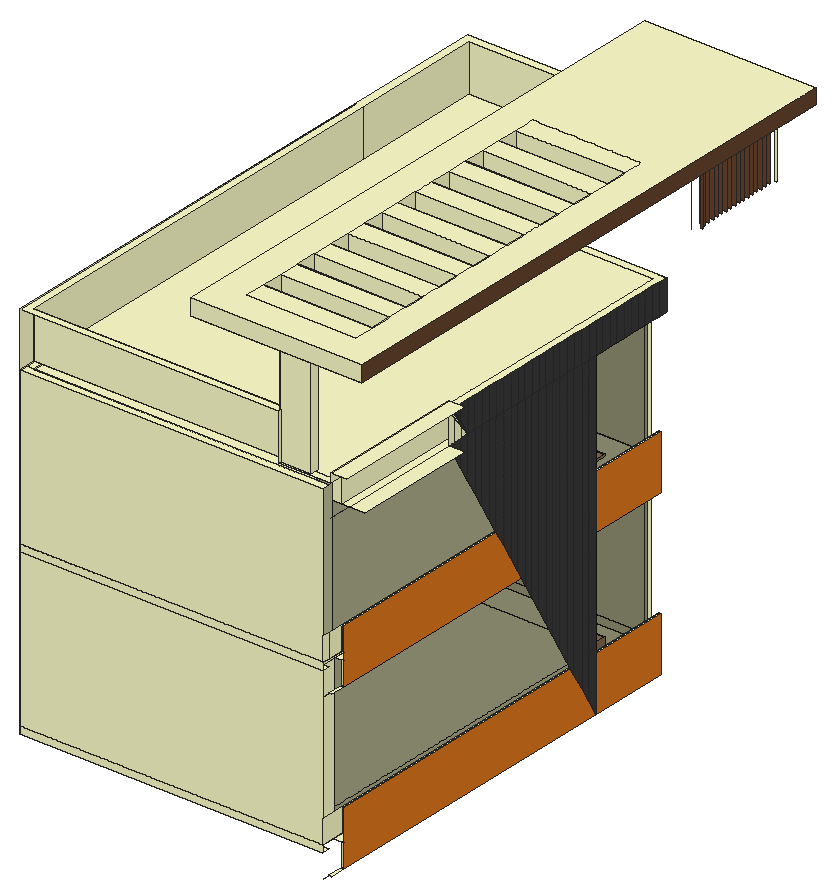
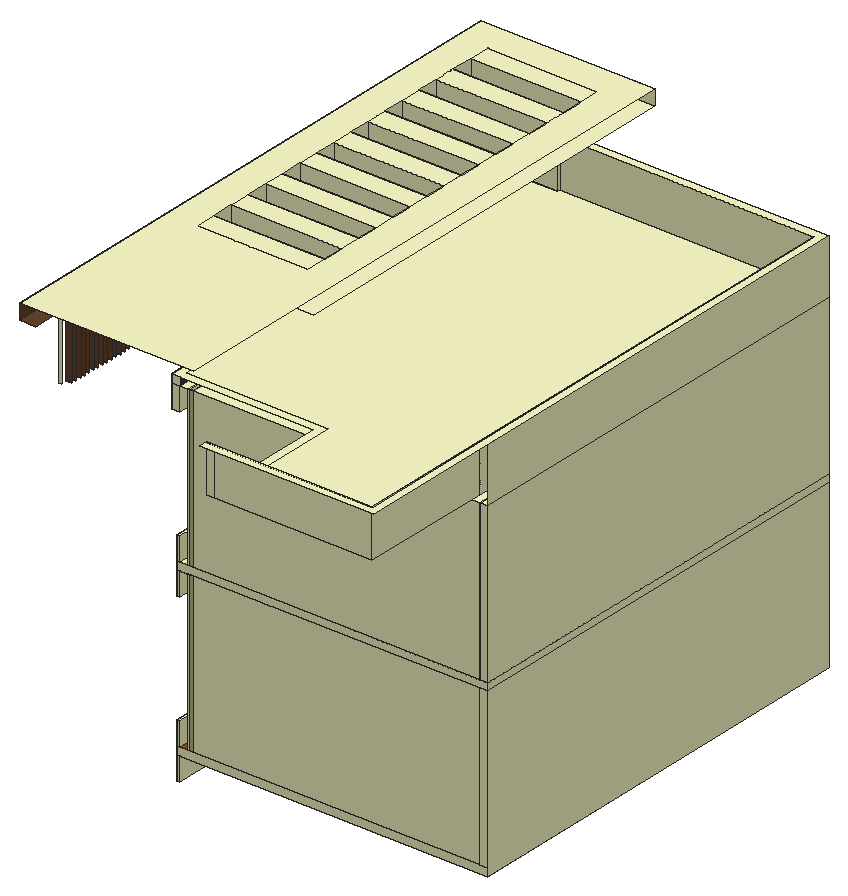
# SketchUp Ruby script. Lengths in inches.
U = 1.inch
M = Sketchup.active_model
def pt(a) = Geom::Point3d.new(a.map { |v| v * U })
def face(e, loops, mat)
  f = e.add_face(loops[0].map { |a| pt(a) })
  loops[1..].each { |l| e.add_face(l.map { |a| pt(a) }).erase! }
  f.material = f.back_material = mat if mat
  f
end
# faces: each face lists its corners as indices into pts; further lists are holes
def faces(e, pts, list, mat = nil) = list.each { |f| face(e, (f[0].is_a?(Array) ? f : [f]).map { |l| l.map { |i| pts[i] } }, mat) }
# xy, xz, yz: faces in a plane at the given z, y or x. An outline is a flat list of corners, or four numbers for a rectangle; further outlines are holes
def ring(l) = l.size == 4 ? [[l[0], l[1]], [l[2], l[1]], [l[2], l[3]], [l[0], l[3]]] : l.each_slice(2).to_a
def flat(e, list, mat, &to3) = list.each { |f| face(e, (f[0].is_a?(Array) ? f : [f]).map { |l| ring(l).map { |u, v| to3.(u, v) } }, mat) }
def xy(e, z, list, mat = nil) = flat(e, list, mat) { |x, y| [x, y, z] }
def xz(e, y, list, mat = nil) = flat(e, list, mat) { |x, z| [x, y, z] }
def yz(e, x, list, mat = nil) = flat(e, list, mat) { |y, z| [x, y, z] }
def lines(e, pts, list) = list.each { |a, b| e.add_line(pt(pts[a]), pt(pts[b])) }
# prism: a flat outline (further loops are holes) pulled along v
def prism(e, loops, v, mat = nil)
  f = face(e, loops, mat); d = Geom::Vector3d.new(v.map { |x| x * U })
  f.pushpull(f.normal.samedirection?(d) ? d.length : -d.length)
end
def box(e, o, s, mat = nil) = prism(e, [[o, [o[0] + s[0], o[1], o[2]], [o[0] + s[0], o[1] + s[1], o[2]], [o[0], o[1] + s[1], o[2]]]], [0, 0, s[2]], mat)
def at(x, y, z, deg = 0) = Geom::Transformation.translation(pt([x, y, z])) * Geom::Transformation.rotation(ORIGIN, Z_AXIS, deg.degrees)
def axes(o, x, y, z) = Geom::Transformation.new([*x, 0, *y, 0, *z, 0, *pt(o).to_a, 1])
def part(name) = M.definitions.add(name)
# library, detail: a bought-in or finely detailed component or shape, given as its bounding box
def library(name, o, s) = part(name).tap { |d| box(d.entities, o, s) }
def detail(e, o, s) = box(e.add_group.entities, o, s)
def put(e, d, t, mat = nil) = e.add_instance(d, t).tap { |i| i.material = mat if mat }
def group(e, t, mat = nil) = e.add_group.tap { |g| g.transformation = t; g.material = mat if mat }.entities
root = M.entities
M.materials.add("Brick_Common_Bond_2K").color = [226, 121, 29]
M.materials.add("E01_Mint_Frost").color = [255, 255, 204]
M.materials.add("Glass_Safety_01").color = [0, 0, 0]
M.materials["Glass_Safety_01"].alpha = 0.25
M.materials.add("M07_Charcoal_Gleam").color = [58, 58, 58]
M.materials.add("Wood_Veneer_15_1K").color = [103, 69, 45]
c1 = library("Sphere Light\#7",[-4.28,-4.28,-4.28],[8.56,8.56,8.56])
c2 = library("Sphere Light\#5",[-3.78,-3.78,-3.78],[7.56,7.56,7.56])
c3 = library("Sphere Light\#6",[-3.67,-3.67,-3.67],[7.34,7.34,7.34])
c4 = library("Sphere Light\#4",[-3.65,-3.65,-3.65],[7.3,7.3,7.3])
c5 = part("Group\#3")
box(c5.entities,[0,0,0],[3,318,120])
c6 = library("Sphere Light\#3",[-3.21,-3.21,-3.21],[6.42,6.42,6.42])
c7 = library("Sphere Light\#2",[-4.11,-4.11,-4.11],[8.22,8.22,8.22])
c8 = library("Sphere Light\#1",[-3.65,-3.65,-3.65],[7.3,7.3,7.3])
c9 = library("Sphere Light",[-3.57,-3.57,-3.57],[7.14,7.14,7.14])
xy(root,492,[[469.07,81.71,471.07,93.71],[469.07,93.71,471.07,399.71]],"E01_Mint_Frost")
xy(root,510,[[235.07,75.71,469.07,81.71],[235.07,81.71,241.07,399.71],[[241.07,81.71,463.07,399.71],[439.31,101.72,440.34,101.92,441.27,102.375,442.0625,103.06,442.65,103.92,442.99,104.91,443.07,105.95,442.87,106.98,442.41,107.92,441.73,108.7,440.87,109.29,439.88,109.63,439.07,109.69,439.07,371.73,439.24,371.72,440.27,371.9,441.22,372.34,442.02,373.01,442.62,373.86,442.98,374.84,443.07,375.88,442.89,376.91,442.45,377.86,441.78,378.66,440.93,379.26,439.95,379.62,438.91,379.71,437.88,379.53,436.93,379.09,436.13,378.42,435.53,377.57,435.17,376.59,435.09,375.71,269.07,375.71,268.9375,376.75,268.54,377.71,267.9,378.54,267.07,379.18,266.11,379.58,265.07,379.71,264.04,379.58,263.07,379.18,262.25,378.54,261.61,377.71,261.21,376.75,261.07,375.71,261.21,374.68,261.61,373.71,262.25,372.89,263.07,372.25,264.04,371.85,265.07,371.71,265.07,109.68,264.43,109.66,263.43,109.36,262.54,108.8125,261.83,108.05,261.33,107.13,261.09,106.11,261.125,105.07,261.43,104.07,261.98,103.18,262.74,102.47,263.66,101.97,264.67,101.73,265.72,101.77,266.72,102.07,267.6,102.62,268.32,103.38,268.81,104.3,269.05,105.3125,269.04,105.71,435.1,105.71,435.08,105.48,435.28,104.45,435.73,103.51,436.42,102.72,437.28,102.14,438.27,101.8]],[463.07,93.71,469.07,399.71],[269.04,105.71,269.02,106.36,268.72,107.36,268.17,108.25,267.41,108.96,266.49,109.45,265.47,109.69,265.07,109.68,265.07,371.71,266.11,371.85,267.07,372.25,267.9,372.89,268.54,373.71,268.9375,374.68,269.07,375.71,435.09,375.71,435.08,375.55,435.26,374.52,435.7,373.57,436.37,372.77,437.22,372.17,438.2,371.8125,439.07,371.73,439.07,109.69,438.84,109.71,437.8125,109.51,436.87,109.05,436.08,108.37,435.5,107.51,435.16,106.52,435.1,105.71]],"E01_Mint_Frost")
xy(root,513,[[439.31,101.72,438.27,101.8,437.28,102.14,436.42,102.72,435.73,103.51,435.28,104.45,435.08,105.48,435.1,105.71,435.16,106.52,435.5,107.51,436.08,108.37,436.87,109.05,437.8125,109.51,438.84,109.71,439.07,109.69,439.88,109.63,440.87,109.29,441.73,108.7,442.41,107.92,442.87,106.98,443.07,105.95,442.99,104.91,442.65,103.92,442.0625,103.06,441.27,102.375,440.34,101.92],[264.67,101.73,263.66,101.97,262.74,102.47,261.98,103.18,261.43,104.07,261.125,105.07,261.09,106.11,261.33,107.13,261.83,108.05,262.54,108.8125,263.43,109.36,264.43,109.66,265.07,109.68,265.47,109.69,266.49,109.45,267.41,108.96,268.17,108.25,268.72,107.36,269.02,106.36,269.04,105.71,269.05,105.3125,268.81,104.3,268.32,103.38,267.6,102.62,266.72,102.07,265.72,101.77],[265.07,371.71,264.04,371.85,263.07,372.25,262.25,372.89,261.61,373.71,261.21,374.68,261.07,375.71,261.21,376.75,261.61,377.71,262.25,378.54,263.07,379.18,264.04,379.58,265.07,379.71,266.11,379.58,267.07,379.18,267.9,378.54,268.54,377.71,268.9375,376.75,269.07,375.71,268.9375,374.68,268.54,373.71,267.9,372.89,267.07,372.25,266.11,371.85],[439.24,371.72,439.07,371.73,438.2,371.8125,437.22,372.17,436.37,372.77,435.7,373.57,435.26,374.52,435.08,375.55,435.09,375.71,435.17,376.59,435.53,377.57,436.13,378.42,436.93,379.09,437.88,379.53,438.91,379.71,439.95,379.62,440.93,379.26,441.78,378.66,442.45,377.86,442.89,376.91,443.07,375.88,442.98,374.84,442.62,373.86,442.02,373.01,441.22,372.34,440.27,371.9]],"E01_Mint_Frost")
xy(root,534,[[469.07,93.71,471.07,399.71]],"E01_Mint_Frost")
xy(root,618,[[469.07,81.71,471.07,93.71],[469.07,93.71,471.07,399.71]],"E01_Mint_Frost")
xy(root,636,[[235.07,75.71,469.07,81.71],[235.07,81.71,241.07,399.71],[[241.07,81.71,463.07,399.71],[439.07,101.71,440.11,101.85,441.07,102.25,441.9,102.89,442.54,103.71,442.9375,104.68,443.07,105.71,442.9375,106.75,442.54,107.71,441.9,108.54,441.07,109.18,440.11,109.58,439.07,109.71,439.07,371.74,439.27,371.72,440.3,371.91,441.24,372.35,442.04,373.03,442.63,373.89,442.98,374.87,443.07,375.91,442.88,376.9375,442.43,377.88,441.76,378.68,440.9,379.27,439.92,379.625,438.875,379.71,437.85,379.52,436.91,379.08,436.11,378.4,435.52,377.54,435.16,376.56,435.09,375.71,269.07,375.71,268.9375,376.75,268.54,377.71,267.9,378.54,267.07,379.18,266.11,379.58,265.07,379.71,264.04,379.58,263.07,379.18,262.25,378.54,261.61,377.71,261.21,376.75,261.07,375.71,261.21,374.68,261.61,373.71,262.25,372.89,263.07,372.25,264.04,371.85,265.07,371.71,265.07,109.69,264.35,109.65,263.35,109.32,262.48,108.76,261.78,107.98,261.3,107.05,261.09,106.03,261.14,104.99,261.46,103.99,262.03,103.12,262.81,102.42,263.74,101.94,264.76,101.73,265.8,101.78,266.79,102.1,267.67,102.67,268.37,103.45,268.84,104.38,269.0625,105.4,269.05,105.71,435.07,105.71,435.21,104.68,435.61,103.71,436.25,102.89,437.07,102.25,438.04,101.85]],[463.07,93.71,469.07,399.71],[269.05,105.71,269.01,106.44,268.68,107.44,268.12,108.3125,267.34,109.01,266.41,109.48,265.39,109.7,265.07,109.69,265.07,371.71,266.11,371.85,267.07,372.25,267.9,372.89,268.54,373.71,268.9375,374.68,269.07,375.71,435.09,375.71,435.08,375.52,435.27,374.49,435.71,373.55,436.39,372.75,437.25,372.16,438.23,371.8,439.07,371.74,439.07,109.71,438.04,109.58,437.07,109.18,436.25,108.54,435.61,107.71,435.21,106.75,435.07,105.71]],"E01_Mint_Frost")
xy(root,637.65,[[439.07,101.71,438.04,101.85,437.07,102.25,436.25,102.89,435.61,103.71,435.21,104.68,435.07,105.71,435.21,106.75,435.61,107.71,436.25,108.54,437.07,109.18,438.04,109.58,439.07,109.71,440.11,109.58,441.07,109.18,441.9,108.54,442.54,107.71,442.9375,106.75,443.07,105.71,442.9375,104.68,442.54,103.71,441.9,102.89,441.07,102.25,440.11,101.85]],"E01_Mint_Frost")
xy(root,639,[[264.76,101.73,263.74,101.94,262.81,102.42,262.03,103.12,261.46,103.99,261.14,104.99,261.09,106.03,261.3,107.05,261.78,107.98,262.48,108.76,263.35,109.32,264.35,109.65,265.07,109.69,265.39,109.7,266.41,109.48,267.34,109.01,268.12,108.3125,268.68,107.44,269.01,106.44,269.05,105.71,269.0625,105.4,268.84,104.38,268.37,103.45,267.67,102.67,266.79,102.1,265.8,101.78],[265.07,371.71,264.04,371.85,263.07,372.25,262.25,372.89,261.61,373.71,261.21,374.68,261.07,375.71,261.21,376.75,261.61,377.71,262.25,378.54,263.07,379.18,264.04,379.58,265.07,379.71,266.11,379.58,267.07,379.18,267.9,378.54,268.54,377.71,268.9375,376.75,269.07,375.71,268.9375,374.68,268.54,373.71,267.9,372.89,267.07,372.25,266.11,371.85],[439.27,371.72,439.07,371.74,438.23,371.8,437.25,372.16,436.39,372.75,435.71,373.55,435.27,374.49,435.08,375.52,435.09,375.71,435.16,376.56,435.52,377.54,436.11,378.4,436.91,379.08,437.85,379.52,438.875,379.71,439.92,379.625,440.9,379.27,441.76,378.68,442.43,377.88,442.88,376.9375,443.07,375.91,442.98,374.87,442.63,373.89,442.04,373.03,441.24,372.35,440.3,371.91]],"E01_Mint_Frost")
xy(root,642,[[235.07,75.71,235.07,399.71,241.07,399.71,241.07,81.71,469.07,81.71,469.07,75.71],[241.07,81.71,461.07,81.71,461.07,93.71,469.07,93.71,469.07,399.71,241.07,399.71]],"E01_Mint_Frost")
xy(root,660,[[469.07,93.71,471.07,399.71]],"E01_Mint_Frost")
xy(root,744,[[469.07,93.71,475.07,399.71],[475.07,93.71,487.07,189.71],[475.07,189.71,475.19,189.71,475.19,207.71,475.07,201.36],[475.07,201.36,475.19,207.71,475.07,207.71]],"E01_Mint_Frost")
xy(root,762,[[235.07,75.71,469.07,81.71],[235.07,81.71,241.07,399.71],[241.07,81.71,241.07,399.71,463.07,399.71,463.07,93.71,461.07,93.71,461.07,81.71],[463.07,93.71,469.07,399.71]],"E01_Mint_Frost")
xy(root,768,[[[434.72,75.71,475.07,75.71,475.07,399.71,367.07,399.71,367.07,501.71,361.07,501.71,361.07,393.71,469.07,393.71,469.07,81.71,458.57,81.71,458.57,77.43,434.72,77.43],[434.57,81.71,458.57,83.43]],[434.57,77.43,434.72,81.71],[434.72,77.43,458.57,81.71],[241.07,81.71,434.57,81.71,434.57,83.43,458.57,83.43,458.57,81.71,469.07,81.71,469.07,393.71,361.07,393.71,361.07,501.71,241.07,501.71],[434.57,81.71,458.57,83.43]],"E01_Mint_Frost")
xy(root,775,[[475.07,75.71,487.07,189.71]],"E01_Mint_Frost")
xy(root,804,[[235.07,75.71,434.72,75.71,434.72,77.43,434.57,77.43,434.57,81.71,241.07,81.71,241.07,501.71,367.07,501.71,367.07,507.71,235.07,507.71]],"E01_Mint_Frost")
xy(root,846,[[[367.07,75.71,499.07,399.71],[391.07,343.24,475.07,359.48],[391.07,310.77,475.07,327.01],[391.07,278.3,475.07,294.54],[391.07,245.83,475.07,262.07],[391.07,180.89,475.07,197.125],[391.07,148.42,475.07,164.66],[391.07,115.95,475.07,132.18],[391.07,213.36,475.07,229.6],[434.57,77.43,458.57,83.43]]],"E01_Mint_Frost")
xy(root,846,[[487.07,399.71,499.07,411.57],[487.07,411.57,499.07,415.79],[487.07,415.79,499.07,420],[485.07,420,499.07,424.21],[481.07,424.21,499.07,428.43],
  [485.07,428.43,499.07,432.64],[481.07,432.64,499.07,436.86],[485.07,436.86,499.07,441.07],[481.07,441.07,499.07,445.29],[485.07,445.29,499.07,449.5],
  [481.07,449.5,499.07,453.71],[485.07,453.71,499.07,457.93],[481.07,457.93,499.07,462.14],[485.07,462.14,499.07,466.36],[481.07,466.36,499.07,470.57],
  [485.07,470.57,499.07,474.79],[481.07,474.79,499.07,479],[485.07,479,499.07,483.21],[481.07,483.21,499.07,487.43],[485.07,487.43,499.07,491.64],
  [487.07,491.64,499.07,495.86],[487.07,495.86,499.07,513.71]],"Wood_Veneer_15_1K")
xy(root,858,[[[367.07,75.71,499.07,513.71],[391.07,99.71,475.07,375.71]],[391.07,99.71,475.07,115.95],[391.07,132.18,475.07,148.42],[391.07,164.66,475.07,180.89],[391.07,197.125,475.07,213.36],
  [391.07,229.6,475.07,245.83],[391.07,262.07,475.07,278.3],[391.07,294.54,475.07,310.77],[391.07,327.01,475.07,343.24],[391.07,359.48,475.07,375.71]],"E01_Mint_Frost")
xz(root,75.71,[[235.07,510,469.07,516],[235.07,516,469.07,636],[235.07,636,469.07,642],[235.07,642,469.07,762],[367.07,846,499.07,858]],"E01_Mint_Frost")
xz(root,77.43,[[434.57,768,434.72,804],[434.72,768,458.57,768,458.57,846,434.57,846,434.57,804,434.72,804]],"E01_Mint_Frost")
xz(root,81.71,[[241.07,516,458.07,636],[461.07,516,463.07,636],[241.07,642,458.07,762],[241.07,768,434.57,804]],"E01_Mint_Frost")
xz(root,83.43,[[434.57,768,458.57,846]],"E01_Mint_Frost")
xz(root,93.71,[[469.07,642,471.07,660],[461.07,744,469.07,762]],"E01_Mint_Frost")
xz(root,115.95,[[391.07,846,475.07,858]],"E01_Mint_Frost")
xz(root,132.18,[[391.07,846,475.07,858]],"E01_Mint_Frost")
xz(root,148.42,[[391.07,846,475.07,858]],"E01_Mint_Frost")
xz(root,164.66,[[391.07,846,475.07,858]],"E01_Mint_Frost")
xz(root,180.89,[[391.07,846,475.07,858]],"E01_Mint_Frost")
xz(root,197.125,[[391.07,846,475.07,858]],"E01_Mint_Frost")
xz(root,213.36,[[391.07,846,475.07,858]],"E01_Mint_Frost")
xz(root,229.6,[[391.07,846,475.07,858]],"E01_Mint_Frost")
xz(root,245.83,[[391.07,846,475.07,858]],"E01_Mint_Frost")
xz(root,262.07,[[391.07,846,475.07,858]],"E01_Mint_Frost")
xz(root,278.3,[[391.07,846,475.07,858]],"E01_Mint_Frost")
xz(root,294.54,[[391.07,846,475.07,858]],"E01_Mint_Frost")
xz(root,310.77,[[391.07,846,475.07,858]],"E01_Mint_Frost")
xz(root,327.01,[[391.07,846,475.07,858]],"E01_Mint_Frost")
xz(root,343.24,[[391.07,846,475.07,858]],"E01_Mint_Frost")
xz(root,359.48,[[391.07,846,475.07,858]],"E01_Mint_Frost")
xz(root,399.71,[[469.07,492,471.07,510],[235.07,510,471.07,516],[235.07,516,241.07,636],[241.07,516,463.07,636],[469.07,516,471.07,534],
  [469.07,618,471.07,636],[235.07,636,471.07,642],[235.07,642,241.07,762],[241.07,642,463.07,762],[469.07,642,471.07,660],
  [469.07,744,475.07,762],[469.07,762,475.07,768]],"E01_Mint_Frost")
xz(root,420,[[485.07,796.83,487.07,846]],"Wood_Veneer_15_1K")
xz(root,424.21,[[481.07,796.9,485.07,846]],"Wood_Veneer_15_1K")
xz(root,428.43,[[481.07,796.96,485.07,846]],"Wood_Veneer_15_1K")
xz(root,432.64,[[481.07,797.03,485.07,846]],"Wood_Veneer_15_1K")
xz(root,436.86,[[481.07,797.09,485.07,846]],"Wood_Veneer_15_1K")
xz(root,441.07,[[481.07,797.16,485.07,846]],"Wood_Veneer_15_1K")
xz(root,445.29,[[481.07,797.22,485.07,846]],"Wood_Veneer_15_1K")
xz(root,449.5,[[481.07,797.29,485.07,846]],"Wood_Veneer_15_1K")
xz(root,453.71,[[481.07,797.35,485.07,846]],"Wood_Veneer_15_1K")
xz(root,457.93,[[481.07,797.42,485.07,846]],"Wood_Veneer_15_1K")
xz(root,462.14,[[481.07,797.48,485.07,846]],"Wood_Veneer_15_1K")
xz(root,466.36,[[481.07,797.55,485.07,846]],"Wood_Veneer_15_1K")
xz(root,470.57,[[481.07,797.61,485.07,846]],"Wood_Veneer_15_1K")
xz(root,474.79,[[481.07,797.68,485.07,846]],"Wood_Veneer_15_1K")
xz(root,479,[[481.07,797.74,485.07,846]],"Wood_Veneer_15_1K")
xz(root,483.21,[[481.07,797.81,485.07,846]],"Wood_Veneer_15_1K")
xz(root,487.43,[[481.07,797.87,485.07,846]],"Wood_Veneer_15_1K")
xz(root,491.64,[[485.07,797.94,487.07,846]],"E01_Mint_Frost")
xz(root,501.71,[[241.07,768,361.07,804],[361.07,768,367.07,804]],"E01_Mint_Frost")
yz(root,235.07,[[75.71,510,399.71,636],[75.71,636,399.71,642],[75.71,642,399.71,762],[75.71,762,399.71,804]],"E01_Mint_Frost")
yz(root,241.07,[[81.71,642,399.71,762],[81.71,768,399.71,804],[399.71,768,501.71,804]],"E01_Mint_Frost")
yz(root,391.07,[[115.95,846,132.18,858],[148.42,846,164.66,858],[180.89,846,197.125,858],[213.36,846,229.6,858],[245.83,846,262.07,858],
  [278.3,846,294.54,858],[310.77,846,327.01,858],[343.24,846,359.48,858]],"E01_Mint_Frost")
yz(root,434.57,[[77.43,768,81.71,804],[81.71,768,81.71,804,77.43,804,77.43,846,83.43,846,83.43,768]],"E01_Mint_Frost")
yz(root,434.72,[[75.71,768,77.43,804]],"E01_Mint_Frost")
yz(root,458.57,[[77.43,768,83.43,846]],"E01_Mint_Frost")
yz(root,461.07,[[81.71,642,93.71,762]],"E01_Mint_Frost")
yz(root,463.07,[[81.71,516,93.71,636]],"E01_Mint_Frost")
yz(root,469.07,[[93.71,492,399.71,510],[75.71,516,93.71,534],[93.71,516,399.71,534],[93.71,618,399.71,636],[75.71,642,81.71,660],
  [81.71,642,93.71,660],[93.71,642,399.71,660],[93.71,744,399.71,762]],"E01_Mint_Frost")
yz(root,471.07,[[93.71,492,399.71,534],[93.71,618,399.71,660]],"Brick_Common_Bond_2K")
yz(root,475.07,[[189.71,744,194.38,744,194.38,766.23,193.3125,768,189.71,768],[194.38,744,201.22,744,201.22,754.82,194.38,766.23],[201.22,744,207.71,744,201.22,754.82],[75.71,768,189.71,775],[189.71,768,193.3125,768,189.71,774],
  [115.95,846,132.18,858],[148.42,846,164.66,858],[180.89,846,197.125,858],[213.36,846,229.6,858],[245.83,846,262.07,858],
  [278.3,846,294.54,858],[310.77,846,327.01,858],[343.24,846,359.48,858]],"E01_Mint_Frost")
yz(root,475.07,[[331.27,496.28,331.27,744,324.42,744,324.42,508.26],[324.42,508.26,324.42,744,317.58,744,317.58,520.23],[317.58,520.23,317.58,744,310.74,744,310.74,532.21],[310.74,532.21,310.74,744,303.89,744,303.89,544.19],[303.89,544.19,303.89,744,297.05,744,297.05,556.17],
  [297.05,556.17,297.05,744,290.2,744,290.2,568.15],[290.2,568.15,290.2,744,283.36,744,283.36,580.125],[283.36,580.125,283.36,744,276.51,744,276.51,592.1],[276.51,592.1,276.51,744,269.67,744,269.67,604.08],[269.67,604.08,269.67,744,262.82,744,262.82,616.06],
  [262.82,616.06,262.82,744,255.98,744,255.98,628.04],[255.98,628.04,255.98,744,249.13,744,249.13,640.01],[249.13,640.01,249.13,744,242.29,744,242.29,651.99],[242.29,651.99,242.29,744,235.45,744,235.45,663.97],[235.45,663.97,235.45,744,228.6,744,228.6,675.95],
  [228.6,675.95,228.6,744,221.76,744,221.76,687.93],[221.76,687.93,221.76,744,214.91,744,214.91,699.9],[214.91,699.9,214.91,744,208.07,744,208.07,711.88],[208.07,711.88,208.07,744,201.22,744,201.22,723.86],[201.22,723.86,201.22,744,194.38,744,194.38,735.84],
  [194.38,735.84,194.38,744,189.71,744],[207.71,744,208.07,744,208.07,768,201.22,768,201.22,754.82],[208.07,744,214.91,768],[214.91,744,221.76,768],[221.76,744,228.6,768],
  [228.6,744,235.45,768],[235.45,744,242.29,768],[242.29,744,249.13,768],[249.13,744,255.98,768],[255.98,744,262.82,768],
  [262.82,744,269.67,768],[269.67,744,276.51,768],[276.51,744,283.36,768],[283.36,744,290.2,768],[290.2,744,297.05,768],
  [297.05,744,303.89,768],[303.89,744,310.74,768],[310.74,744,317.58,768],[317.58,744,324.42,768],[324.42,744,331.27,768],
  [331.27,744,338.11,768],[338.11,744,344.96,768],[344.96,744,351.8,768],[351.8,744,358.65,768],[358.65,744,365.49,768],
  [365.49,744,372.34,768],[372.34,744,379.18,768],[379.18,744,386.03,768],[386.03,744,392.87,768],[392.87,744,399.71,768],
  [201.22,754.82,201.22,768,194.38,768,194.38,766.23],[194.38,766.23,194.38,768,193.3125,768]],"M07_Charcoal_Gleam")
yz(root,475.19,[[207.71,743.54,207.71,744,207.45,744],[207.45,744,207.71,744,189.71,775]],"E01_Mint_Frost")
yz(root,499.07,[[75.71,846,513.71,858]],"Wood_Veneer_15_1K")
p = [[264.67,101.73,510],[263.66,101.97,510],[263.66,101.97,513],[264.67,101.73,513],[265.72,101.77,510],[265.72,101.77,513],
  [439.31,101.72,510],[438.27,101.8,510],[438.27,101.8,513],[439.31,101.72,513],[440.34,101.92,510],[440.34,101.92,513],
  [266.72,102.07,510],[266.72,102.07,513],[437.28,102.14,510],[437.28,102.14,513],[441.27,102.375,510],[441.27,102.375,513],
  [262.74,102.47,510],[262.74,102.47,513],[267.6,102.62,510],[267.6,102.62,513],[436.42,102.72,510],[436.42,102.72,513],
  [442.0625,103.06,510],[442.0625,103.06,513],[261.98,103.18,510],[261.98,103.18,513],[268.32,103.38,510],[268.32,103.38,513],
  [435.73,103.51,510],[435.73,103.51,513],[442.65,103.92,510],[442.65,103.92,513],[261.43,104.07,510],[261.43,104.07,513],
  [268.81,104.3,510],[268.81,104.3,513],[435.28,104.45,510],[435.28,104.45,513],[442.99,104.91,510],[442.99,104.91,513],
  [261.125,105.07,510],[261.125,105.07,513],[269.05,105.3125,510],[269.05,105.3125,513],[435.08,105.48,510],[435.08,105.48,513],
  [443.07,105.95,510],[443.07,105.95,513],[261.09,106.11,510],[261.09,106.11,513],[269.04,105.71,510],[269.04,105.71,513],
  [435.1,105.71,510],[435.1,105.71,513],[269.02,106.36,510],[269.02,106.36,513],[435.16,106.52,510],[435.16,106.52,513],
  [442.87,106.98,510],[442.87,106.98,513],[261.33,107.13,510],[261.33,107.13,513],[268.72,107.36,510],[268.72,107.36,513],
  [435.5,107.51,510],[435.5,107.51,513],[442.41,107.92,510],[442.41,107.92,513],[261.83,108.05,510],[261.83,108.05,513],
  [268.17,108.25,510],[268.17,108.25,513],[436.08,108.37,510],[436.08,108.37,513],[441.73,108.7,510],[441.73,108.7,513],
  [262.54,108.8125,510],[262.54,108.8125,513],[267.41,108.96,510],[267.41,108.96,513],[436.87,109.05,510],[436.87,109.05,513],
  [440.87,109.29,510],[440.87,109.29,513],[263.43,109.36,510],[263.43,109.36,513],[266.49,109.45,510],[266.49,109.45,513],
  [437.8125,109.51,510],[437.8125,109.51,513],[439.88,109.63,510],[439.88,109.63,513],[264.43,109.66,510],[264.43,109.66,513],
  [265.47,109.69,510],[265.47,109.69,513],[438.84,109.71,510],[438.84,109.71,513],[439.07,109.69,510],[439.07,109.69,513],
  [265.07,109.68,510],[265.07,109.68,513],[265.07,371.71,510],[264.04,371.85,510],[264.04,371.85,513],[265.07,371.71,513],
  [266.11,371.85,510],[266.11,371.85,513],[439.07,371.73,510],[438.2,371.8125,510],[438.2,371.8125,513],[439.07,371.73,513],
  [439.24,371.72,510],[439.24,371.72,513],[440.27,371.9,510],[440.27,371.9,513],[437.22,372.17,510],[437.22,372.17,513],
  [263.07,372.25,510],[263.07,372.25,513],[267.07,372.25,510],[267.07,372.25,513],[441.22,372.34,510],[441.22,372.34,513],
  [436.37,372.77,510],[436.37,372.77,513],[262.25,372.89,510],[262.25,372.89,513],[267.9,372.89,510],[267.9,372.89,513],
  [442.02,373.01,510],[442.02,373.01,513],[435.7,373.57,510],[435.7,373.57,513],[261.61,373.71,510],[261.61,373.71,513],
  [268.54,373.71,510],[268.54,373.71,513],[442.62,373.86,510],[442.62,373.86,513],[435.26,374.52,510],[435.26,374.52,513],
  [261.21,374.68,510],[261.21,374.68,513],[268.9375,374.68,510],[268.9375,374.68,513],[442.98,374.84,510],[442.98,374.84,513],
  [435.08,375.55,510],[435.08,375.55,513],[261.07,375.71,510],[261.07,375.71,513],[269.07,375.71,510],[269.07,375.71,513],
  [443.07,375.88,510],[443.07,375.88,513],[435.09,375.71,510],[435.09,375.71,513],[261.21,376.75,510],[261.21,376.75,513],
  [268.9375,376.75,510],[268.9375,376.75,513],[435.17,376.59,510],[435.17,376.59,513],[442.89,376.91,510],[442.89,376.91,513],
  [435.53,377.57,510],[435.53,377.57,513],[261.61,377.71,510],[261.61,377.71,513],[268.54,377.71,510],[268.54,377.71,513],
  [442.45,377.86,510],[442.45,377.86,513],[436.13,378.42,510],[436.13,378.42,513],[262.25,378.54,510],[262.25,378.54,513],
  [267.9,378.54,510],[267.9,378.54,513],[441.78,378.66,510],[441.78,378.66,513],[436.93,379.09,510],[436.93,379.09,513],
  [263.07,379.18,510],[263.07,379.18,513],[267.07,379.18,510],[267.07,379.18,513],[440.93,379.26,510],[440.93,379.26,513],
  [437.88,379.53,510],[437.88,379.53,513],[264.04,379.58,510],[264.04,379.58,513],[266.11,379.58,510],[266.11,379.58,513],
  [439.95,379.62,510],[439.95,379.62,513],[438.91,379.71,510],[438.91,379.71,513],[265.07,379.71,510],[265.07,379.71,513],
  [264.76,101.73,636],[263.74,101.94,636],[263.74,101.94,639],[264.76,101.73,639],[265.8,101.78,636],[265.8,101.78,639],
  [439.07,101.71,636],[438.04,101.85,636],[438.04,101.85,637.65],[439.07,101.71,637.65],[440.11,101.85,636],[440.11,101.85,637.65],
  [266.79,102.1,636],[266.79,102.1,639],[262.81,102.42,636],[262.81,102.42,639],[437.07,102.25,636],[437.07,102.25,637.65],
  [441.07,102.25,636],[441.07,102.25,637.65],[267.67,102.67,636],[267.67,102.67,639],[436.25,102.89,636],[436.25,102.89,637.65],
  [441.9,102.89,636],[441.9,102.89,637.65],[262.03,103.12,636],[262.03,103.12,639],[268.37,103.45,636],[268.37,103.45,639],
  [435.61,103.71,636],[435.61,103.71,637.65],[442.54,103.71,636],[442.54,103.71,637.65],[261.46,103.99,636],[261.46,103.99,639],
  [268.84,104.38,636],[268.84,104.38,639],[435.21,104.68,636],[435.21,104.68,637.65],[442.9375,104.68,636],[442.9375,104.68,637.65],
  [261.14,104.99,636],[261.14,104.99,639],[269.0625,105.4,636],[269.0625,105.4,639],[435.07,105.71,636],[435.07,105.71,637.65],
  [443.07,105.71,636],[443.07,105.71,637.65],[261.09,106.03,636],[261.09,106.03,639],[269.05,105.71,636],[269.05,105.71,639],
  [269.01,106.44,636],[269.01,106.44,639],[435.21,106.75,636],[435.21,106.75,637.65],[442.9375,106.75,636],[442.9375,106.75,637.65],
  [261.3,107.05,636],[261.3,107.05,639],[268.68,107.44,636],[268.68,107.44,639],[435.61,107.71,636],[435.61,107.71,637.65],
  [442.54,107.71,636],[442.54,107.71,637.65],[261.78,107.98,636],[261.78,107.98,639],[268.12,108.3125,636],[268.12,108.3125,639],
  [436.25,108.54,636],[436.25,108.54,637.65],[441.9,108.54,636],[441.9,108.54,637.65],[262.48,108.76,636],[262.48,108.76,639],
  [267.34,109.01,636],[267.34,109.01,639],[437.07,109.18,636],[437.07,109.18,637.65],[441.07,109.18,636],[441.07,109.18,637.65],
  [263.35,109.32,636],[263.35,109.32,639],[266.41,109.48,636],[266.41,109.48,639],[438.04,109.58,636],[438.04,109.58,637.65],
  [440.11,109.58,636],[440.11,109.58,637.65],[264.35,109.65,636],[264.35,109.65,639],[265.39,109.7,636],[265.39,109.7,639],
  [265.07,109.69,636],[265.07,109.69,639],[439.07,109.71,636],[439.07,109.71,637.65],[265.07,371.71,636],[264.04,371.85,636],
  [264.04,371.85,639],[265.07,371.71,639],[266.11,371.85,636],[266.11,371.85,639],[439.07,371.74,636],[438.23,371.8,636],
  [438.23,371.8,639],[439.07,371.74,639],[439.27,371.72,636],[439.27,371.72,639],[440.3,371.91,636],[440.3,371.91,639],
  [437.25,372.16,636],[437.25,372.16,639],[263.07,372.25,636],[263.07,372.25,639],[267.07,372.25,636],[267.07,372.25,639],
  [441.24,372.35,636],[441.24,372.35,639],[436.39,372.75,636],[436.39,372.75,639],[262.25,372.89,636],[262.25,372.89,639],
  [267.9,372.89,636],[267.9,372.89,639],[442.04,373.03,636],[442.04,373.03,639],[435.71,373.55,636],[435.71,373.55,639],
  [261.61,373.71,636],[261.61,373.71,639],[268.54,373.71,636],[268.54,373.71,639],[442.63,373.89,636],[442.63,373.89,639],
  [435.27,374.49,636],[435.27,374.49,639],[261.21,374.68,636],[261.21,374.68,639],[268.9375,374.68,636],[268.9375,374.68,639],
  [442.98,374.87,636],[442.98,374.87,639],[435.08,375.52,636],[435.08,375.52,639],[261.07,375.71,636],[261.07,375.71,639],
  [269.07,375.71,636],[269.07,375.71,639],[443.07,375.91,636],[443.07,375.91,639],[435.09,375.71,636],[435.09,375.71,639],
  [261.21,376.75,636],[261.21,376.75,639],[268.9375,376.75,636],[268.9375,376.75,639],[435.16,376.56,636],[435.16,376.56,639],
  [442.88,376.9375,636],[442.88,376.9375,639],[435.52,377.54,636],[435.52,377.54,639],[261.61,377.71,636],[261.61,377.71,639],
  [268.54,377.71,636],[268.54,377.71,639],[442.43,377.88,636],[442.43,377.88,639],[436.11,378.4,636],[436.11,378.4,639],
  [262.25,378.54,636],[262.25,378.54,639],[267.9,378.54,636],[267.9,378.54,639],[441.76,378.68,636],[441.76,378.68,639],
  [436.91,379.08,636],[436.91,379.08,639],[263.07,379.18,636],[263.07,379.18,639],[267.07,379.18,636],[267.07,379.18,639],
  [440.9,379.27,636],[440.9,379.27,639],[437.85,379.52,636],[437.85,379.52,639],[264.04,379.58,636],[264.04,379.58,639],
  [266.11,379.58,636],[266.11,379.58,639],[439.92,379.625,636],[439.92,379.625,639],[438.875,379.71,636],[438.875,379.71,639],
  [265.07,379.71,636],[265.07,379.71,639],[475.07,189.71,770],[475.19,207.71,744],[475.07,189.71,768],[475.07,189.71,775],
  [475.07,189.71,774],[475.19,189.71,775],[481.07,415.79,796.77],[481.07,415.79,846],[463.07,399.71,642],[463.07,153.71,642],
  [471.07,93.71,642],[471.07,75.71,642],[469.07,93.71,762],[471.07,93.71,762],[475.19,207.71,712.5],[475.19,207.71,743.54],
  [458.07,81.71,516],[461.07,81.71,516],[469.07,93.71,636],[471.07,93.71,636],[469.07,93.71,510],[471.07,93.71,510],
  [469.07,81.71,618],[469.07,75.71,618],[463.07,399.71,516],[463.07,153.71,516],[469.07,81.71,492],[469.07,75.71,492],
  [487.07,189.71,768],[487.07,189.71,770],[487.07,189.71,774],[475.07,192.71,768],[475.19,192.71,768],[265.07,105.71,762],
  [265.07,375.71,762],[439.07,375.71,762],[439.07,105.71,762],[475.07,93.71,744],[475.07,75.71,744]]
faces(root,p,[[0,1,2,3],[4,0,3,5],[6,7,8,9],[10,6,9,11],[12,4,5,13],[7,14,15,8],[16,10,11,17],[1,18,19,2],
  [20,12,13,21],[14,22,23,15],[24,16,17,25],[18,26,27,19],[28,20,21,29],[22,30,31,23],[32,24,25,33],[26,34,35,27],
  [36,28,29,37],[30,38,39,31],[40,32,33,41],[34,42,43,35],[44,36,37,45],[38,46,47,39],[48,40,41,49],[42,50,51,43],
  [52,44,45,53],[46,54,55,47],[56,52,53,57],[54,58,59,55],[60,48,49,61],[50,62,63,51],[64,56,57,65],[58,66,67,59],
  [68,60,61,69],[62,70,71,63],[72,64,65,73],[66,74,75,67],[76,68,69,77],[70,78,79,71],[80,72,73,81],[74,82,83,75],
  [84,76,77,85],[78,86,87,79],[88,80,81,89],[82,90,91,83],[92,84,85,93],[86,94,95,87],[96,88,89,97],[90,98,99,91],
  [100,92,93,101],[94,102,103,95],[102,96,97,103],[98,100,101,99],[104,105,106,107],[108,104,107,109],[110,111,112,113],[114,110,113,115],
  [116,114,115,117],[111,118,119,112],[105,120,121,106],[122,108,109,123],[124,116,117,125],[118,126,127,119],[120,128,129,121],[130,122,123,131],
  [132,124,125,133],[126,134,135,127],[128,136,137,129],[138,130,131,139],[140,132,133,141],[134,142,143,135],[136,144,145,137],[146,138,139,147],
  [148,140,141,149],[142,150,151,143],[144,152,153,145],[154,146,147,155],[156,148,149,157],[150,158,159,151],[152,160,161,153],[162,154,155,163],
  [158,164,165,159],[166,156,157,167],[164,168,169,165],[160,170,171,161],[172,162,163,173],[174,166,167,175],[168,176,177,169],[170,178,179,171],
  [180,172,173,181],[182,174,175,183],[176,184,185,177],[178,186,187,179],[188,180,181,189],[190,182,183,191],[184,192,193,185],[186,194,195,187],
  [196,188,189,197],[198,190,191,199],[192,200,201,193],[194,202,203,195],[202,196,197,203],[200,198,199,201],[204,205,206,207],[208,204,207,209],
  [210,211,212,213],[214,210,213,215],[216,208,209,217],[205,218,219,206],[211,220,221,212],[222,214,215,223],[224,216,217,225],[220,226,227,221],
  [228,222,223,229],[218,230,231,219],[232,224,225,233],[226,234,235,227],[236,228,229,237],[230,238,239,231],[240,232,233,241],[234,242,243,235],
  [244,236,237,245],[238,246,247,239],[248,240,241,249],[242,250,251,243],[252,244,245,253],[246,254,255,247],[256,248,249,257],[258,256,257,259],
  [250,260,261,251],[262,252,253,263],[254,264,265,255],[266,258,259,267],[260,268,269,261],[270,262,263,271],[264,272,273,265],[274,266,267,275],
  [268,276,277,269],[278,270,271,279],[272,280,281,273],[282,274,275,283],[276,284,285,277],[286,278,279,287],[280,288,289,281],[290,282,283,291],
  [284,292,293,285],[294,286,287,295],[288,296,297,289],[298,290,291,299],[296,300,301,297],[292,302,303,293],[302,294,295,303],[300,298,299,301],
  [304,305,306,307],[308,304,307,309],[310,311,312,313],[314,310,313,315],[316,314,315,317],[311,318,319,312],[305,320,321,306],[322,308,309,323],
  [324,316,317,325],[318,326,327,319],[320,328,329,321],[330,322,323,331],[332,324,325,333],[326,334,335,327],[328,336,337,329],[338,330,331,339],
  [340,332,333,341],[334,342,343,335],[336,344,345,337],[346,338,339,347],[348,340,341,349],[342,350,351,343],[344,352,353,345],[354,346,347,355],
  [356,348,349,357],[350,358,359,351],[352,360,361,353],[362,354,355,363],[358,364,365,359],[366,356,357,367],[364,368,369,365],[360,370,371,361],
  [372,362,363,373],[374,366,367,375],[368,376,377,369],[370,378,379,371],[380,372,373,381],[382,374,375,383],[376,384,385,377],[378,386,387,379],
  [388,380,381,389],[390,382,383,391],[384,392,393,385],[386,394,395,387],[396,388,389,397],[398,390,391,399],[392,400,401,393],[394,402,403,395],
  [402,396,397,403],[400,398,399,401],[404,405,406],[407,405,404,408],[407,409,405]],"E01_Mint_Frost")
lines(root,p,[[410,411],[412,413],[414,415],[416,417],[418,419],[420,421],[422,423],[424,425],[426,427],[428,429],[430,431],[432,406],
  [433,404],[434,408],[435,436],[437,438],[438,439],[439,440],[440,437],[441,442]])
put(root,c1,at(439.21,375.11,513),"E01_Mint_Frost")
put(root,c2,at(265.13,106.05,513),"E01_Mint_Frost")
put(root,c3,at(265.53,375.54,513),"E01_Mint_Frost")
put(root,c4,at(439.3,105.8,513),"E01_Mint_Frost")
put(root,c5,at(458.07,81.71,516),"Glass_Safety_01")
put(root,c6,at(438.68,106.1,637.65),"E01_Mint_Frost")
put(root,c7,at(438.97,376.05,639),"E01_Mint_Frost")
put(root,c8,at(265.125,375.6,639),"E01_Mint_Frost")
put(root,c9,at(264.5625,105.61,639),"E01_Mint_Frost")
put(root,c5,at(458.07,81.71,642),"Glass_Safety_01")
